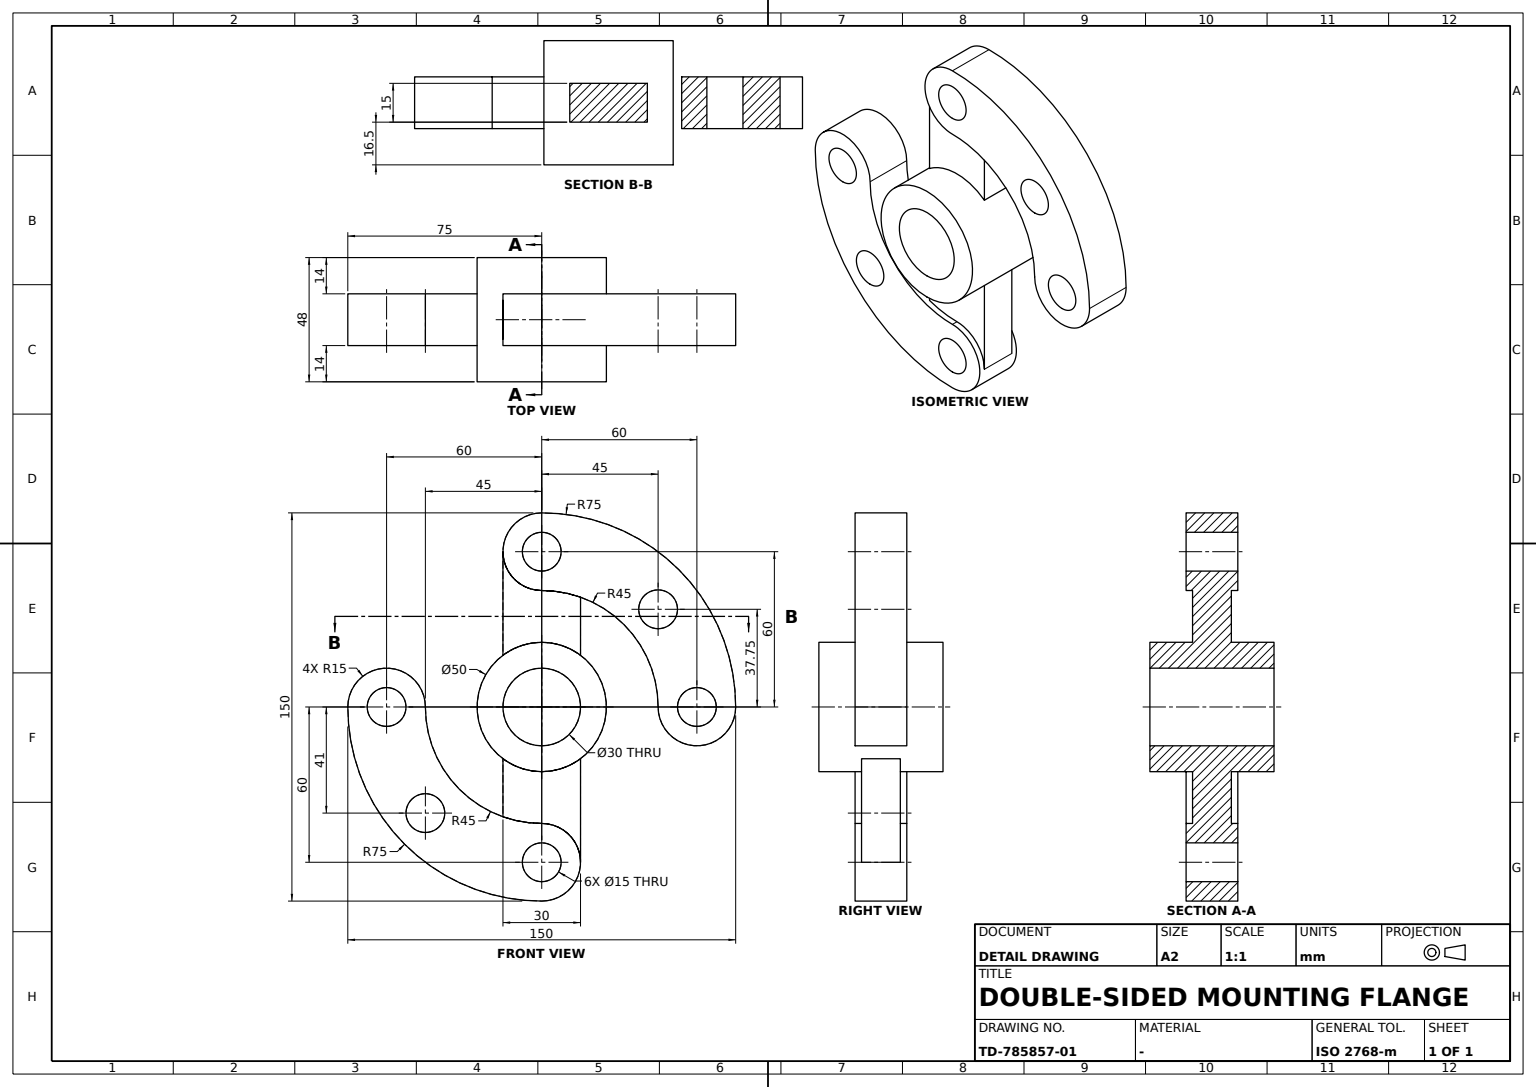
ISO-10303-21;
HEADER;
FILE_DESCRIPTION((''),'2;1');
FILE_NAME('','',(''),(''),'','','');
FILE_SCHEMA(('AUTOMOTIVE_DESIGN'));
ENDSEC;
DATA;
#1=APPLICATION_CONTEXT('');
#2=PRODUCT_CONTEXT('',#1,'mechanical');
#3=PRODUCT('','','',(#2));
#4=PRODUCT_DEFINITION_FORMATION('','',#3);
#5=PRODUCT_DEFINITION_CONTEXT('',#1,'design');
#6=PRODUCT_DEFINITION('','',#4,#5);
#7=PRODUCT_DEFINITION_SHAPE('','',#6);
#8=(LENGTH_UNIT()NAMED_UNIT(*)SI_UNIT(.MILLI.,.METRE.));
#9=(NAMED_UNIT(*)PLANE_ANGLE_UNIT()SI_UNIT($,.RADIAN.));
#10=(NAMED_UNIT(*)SI_UNIT($,.STERADIAN.)SOLID_ANGLE_UNIT());
#11=UNCERTAINTY_MEASURE_WITH_UNIT(LENGTH_MEASURE(0.005),#8,'distance_accuracy_value','');
#12=(GEOMETRIC_REPRESENTATION_CONTEXT(3)GLOBAL_UNCERTAINTY_ASSIGNED_CONTEXT((#11))GLOBAL_UNIT_ASSIGNED_CONTEXT((#8,#9,#10))REPRESENTATION_CONTEXT('',''));
#13=CARTESIAN_POINT('',(-10.,-60.,-7.5));
#14=VERTEX_POINT('',#13);
#15=CARTESIAN_POINT('',(-10.,-60.,0.));
#16=DIRECTION('',(1.,0.,0.));
#17=DIRECTION('',(0.,0.,-1.));
#18=AXIS2_PLACEMENT_3D('',#15,#16,#17);
#19=CIRCLE('',#18,7.5);
#20=EDGE_CURVE('',#14,#14,#19,.T.);
#21=ORIENTED_EDGE('',*,*,#20,.F.);
#22=EDGE_LOOP('',(#21));
#23=FACE_BOUND('',#22,.T.);
#24=CARTESIAN_POINT('',(10.,-60.,-7.5));
#25=VERTEX_POINT('',#24);
#26=CARTESIAN_POINT('',(10.,-60.,0.));
#27=AXIS2_PLACEMENT_3D('',#26,#16,#17);
#28=CIRCLE('',#27,7.5);
#29=EDGE_CURVE('',#25,#25,#28,.T.);
#30=ORIENTED_EDGE('',*,*,#29,.T.);
#31=EDGE_LOOP('',(#30));
#32=FACE_BOUND('',#31,.T.);
#33=CARTESIAN_POINT('',(0.,-60.,0.));
#34=DIRECTION('',(0.,1.,0.));
#35=AXIS2_PLACEMENT_3D('',#33,#16,#34);
#36=CYLINDRICAL_SURFACE('',#35,7.5);
#37=ADVANCED_FACE('',(#23,#32),#36,.F.);
#38=CARTESIAN_POINT('',(-10.,-45.,-48.498329));
#39=VERTEX_POINT('',#38);
#40=CARTESIAN_POINT('',(-10.,-45.,-40.998329));
#41=AXIS2_PLACEMENT_3D('',#40,#16,#17);
#42=CIRCLE('',#41,7.5);
#43=EDGE_CURVE('',#39,#39,#42,.T.);
#44=ORIENTED_EDGE('',*,*,#43,.T.);
#45=EDGE_LOOP('',(#44));
#46=FACE_BOUND('',#45,.T.);
#47=CARTESIAN_POINT('',(-10.,0.,-67.5));
#48=VERTEX_POINT('',#47);
#49=CARTESIAN_POINT('',(-10.,0.,-60.));
#50=AXIS2_PLACEMENT_3D('',#49,#16,#17);
#51=CIRCLE('',#50,7.5);
#52=EDGE_CURVE('',#48,#48,#51,.T.);
#53=ORIENTED_EDGE('',*,*,#52,.T.);
#54=EDGE_LOOP('',(#53));
#55=FACE_BOUND('',#54,.T.);
#56=CARTESIAN_POINT('',(-10.,-45.,0.));
#57=VERTEX_POINT('',#56);
#58=CARTESIAN_POINT('',(-10.,0.,-45.));
#59=VERTEX_POINT('',#58);
#60=CARTESIAN_POINT('',(-10.,0.,0.));
#61=AXIS2_PLACEMENT_3D('',#60,#16,#17);
#62=CIRCLE('',#61,45.);
#63=EDGE_CURVE('',#57,#59,#62,.T.);
#64=ORIENTED_EDGE('',*,*,#63,.T.);
#65=CARTESIAN_POINT('',(-10.,0.,-75.));
#66=VERTEX_POINT('',#65);
#67=CIRCLE('',#50,15.);
#68=EDGE_CURVE('',#66,#59,#67,.T.);
#69=ORIENTED_EDGE('',*,*,#68,.F.);
#70=CARTESIAN_POINT('',(-10.,-75.,0.));
#71=VERTEX_POINT('',#70);
#72=CIRCLE('',#61,75.);
#73=EDGE_CURVE('',#71,#66,#72,.T.);
#74=ORIENTED_EDGE('',*,*,#73,.F.);
#75=CIRCLE('',#18,15.);
#76=EDGE_CURVE('',#57,#71,#75,.T.);
#77=ORIENTED_EDGE('',*,*,#76,.F.);
#78=EDGE_LOOP('',(#64,#69,#74,#77));
#79=FACE_BOUND('',#78,.T.);
#80=ORIENTED_EDGE('',*,*,#20,.T.);
#81=EDGE_LOOP('',(#80));
#82=FACE_BOUND('',#81,.T.);
#83=AXIS2_PLACEMENT_3D('',#60,#16,#34);
#84=PLANE('',#83);
#85=ADVANCED_FACE('',(#46,#55,#79,#82),#84,.F.);
#86=CARTESIAN_POINT('',(-10.,60.,-7.5));
#87=VERTEX_POINT('',#86);
#88=CARTESIAN_POINT('',(-10.,60.,0.));
#89=AXIS2_PLACEMENT_3D('',#88,#16,#17);
#90=CIRCLE('',#89,7.5);
#91=EDGE_CURVE('',#87,#87,#90,.T.);
#92=ORIENTED_EDGE('',*,*,#91,.F.);
#93=EDGE_LOOP('',(#92));
#94=FACE_BOUND('',#93,.T.);
#95=CARTESIAN_POINT('',(10.,60.,-7.5));
#96=VERTEX_POINT('',#95);
#97=CARTESIAN_POINT('',(10.,60.,0.));
#98=AXIS2_PLACEMENT_3D('',#97,#16,#17);
#99=CIRCLE('',#98,7.5);
#100=EDGE_CURVE('',#96,#96,#99,.T.);
#101=ORIENTED_EDGE('',*,*,#100,.T.);
#102=EDGE_LOOP('',(#101));
#103=FACE_BOUND('',#102,.T.);
#104=CARTESIAN_POINT('',(0.,60.,0.));
#105=AXIS2_PLACEMENT_3D('',#104,#16,#34);
#106=CYLINDRICAL_SURFACE('',#105,7.5);
#107=ADVANCED_FACE('',(#94,#103),#106,.F.);
#108=CARTESIAN_POINT('',(24.,0.,-25.));
#109=VERTEX_POINT('',#108);
#110=CARTESIAN_POINT('',(24.,0.,0.));
#111=AXIS2_PLACEMENT_3D('',#110,#16,#17);
#112=CIRCLE('',#111,25.);
#113=EDGE_CURVE('',#109,#109,#112,.T.);
#114=ORIENTED_EDGE('',*,*,#113,.F.);
#115=EDGE_LOOP('',(#114));
#116=FACE_BOUND('',#115,.T.);
#117=CARTESIAN_POINT('',(-7.5,15.,20.));
#118=VERTEX_POINT('',#117);
#119=CARTESIAN_POINT('',(-7.5,-15.,20.));
#120=VERTEX_POINT('',#119);
#121=CARTESIAN_POINT('',(-7.5,0.,0.));
#122=AXIS2_PLACEMENT_3D('',#121,#16,#17);
#123=CIRCLE('',#122,25.);
#124=EDGE_CURVE('',#118,#120,#123,.T.);
#125=ORIENTED_EDGE('',*,*,#124,.F.);
#126=CARTESIAN_POINT('',(7.5,15.,20.));
#127=VERTEX_POINT('',#126);
#128=VECTOR('',#16,1000.);
#129=LINE('',#117,#128);
#130=EDGE_CURVE('',#118,#127,#129,.T.);
#131=ORIENTED_EDGE('',*,*,#130,.T.);
#132=CARTESIAN_POINT('',(7.5,-15.,20.));
#133=VERTEX_POINT('',#132);
#134=CARTESIAN_POINT('',(7.5,0.,0.));
#135=AXIS2_PLACEMENT_3D('',#134,#16,#17);
#136=CIRCLE('',#135,25.);
#137=EDGE_CURVE('',#127,#133,#136,.T.);
#138=ORIENTED_EDGE('',*,*,#137,.T.);
#139=LINE('',#119,#128);
#140=EDGE_CURVE('',#120,#133,#139,.T.);
#141=ORIENTED_EDGE('',*,*,#140,.F.);
#142=EDGE_LOOP('',(#125,#131,#138,#141));
#143=FACE_BOUND('',#142,.T.);
#144=CARTESIAN_POINT('',(-7.5,-15.,-20.));
#145=VERTEX_POINT('',#144);
#146=CARTESIAN_POINT('',(7.5,-15.,-20.));
#147=VERTEX_POINT('',#146);
#148=LINE('',#144,#128);
#149=EDGE_CURVE('',#145,#147,#148,.T.);
#150=ORIENTED_EDGE('',*,*,#149,.T.);
#151=CARTESIAN_POINT('',(7.5,15.,-20.));
#152=VERTEX_POINT('',#151);
#153=EDGE_CURVE('',#147,#152,#136,.T.);
#154=ORIENTED_EDGE('',*,*,#153,.T.);
#155=CARTESIAN_POINT('',(-7.5,15.,-20.));
#156=VERTEX_POINT('',#155);
#157=LINE('',#155,#128);
#158=EDGE_CURVE('',#156,#152,#157,.T.);
#159=ORIENTED_EDGE('',*,*,#158,.F.);
#160=EDGE_CURVE('',#145,#156,#123,.T.);
#161=ORIENTED_EDGE('',*,*,#160,.F.);
#162=EDGE_LOOP('',(#150,#154,#159,#161));
#163=FACE_BOUND('',#162,.T.);
#164=CARTESIAN_POINT('',(-24.,0.,-25.));
#165=VERTEX_POINT('',#164);
#166=CARTESIAN_POINT('',(-24.,0.,0.));
#167=AXIS2_PLACEMENT_3D('',#166,#16,#17);
#168=CIRCLE('',#167,25.);
#169=EDGE_CURVE('',#165,#165,#168,.T.);
#170=ORIENTED_EDGE('',*,*,#169,.T.);
#171=EDGE_LOOP('',(#170));
#172=FACE_BOUND('',#171,.T.);
#173=CARTESIAN_POINT('',(0.,0.,0.));
#174=AXIS2_PLACEMENT_3D('',#173,#16,#34);
#175=CYLINDRICAL_SURFACE('',#174,25.);
#176=ADVANCED_FACE('',(#116,#143,#163,#172),#175,.T.);
#177=CARTESIAN_POINT('',(7.5,15.,42.426407));
#178=VERTEX_POINT('',#177);
#179=CARTESIAN_POINT('',(7.5,0.,45.));
#180=VERTEX_POINT('',#179);
#181=CIRCLE('',#135,45.);
#182=EDGE_CURVE('',#178,#180,#181,.T.);
#183=ORIENTED_EDGE('',*,*,#182,.T.);
#184=CARTESIAN_POINT('',(7.5,-15.,60.));
#185=VERTEX_POINT('',#184);
#186=CARTESIAN_POINT('',(7.5,0.,60.));
#187=AXIS2_PLACEMENT_3D('',#186,#16,#17);
#188=CIRCLE('',#187,15.);
#189=EDGE_CURVE('',#185,#180,#188,.T.);
#190=ORIENTED_EDGE('',*,*,#189,.F.);
#191=CARTESIAN_POINT('',(7.5,-15.,0.));
#192=DIRECTION('',(0.,0.,1.));
#193=VECTOR('',#192,1000.);
#194=LINE('',#191,#193);
#195=EDGE_CURVE('',#133,#185,#194,.T.);
#196=ORIENTED_EDGE('',*,*,#195,.F.);
#197=ORIENTED_EDGE('',*,*,#137,.F.);
#198=CARTESIAN_POINT('',(7.5,15.,0.));
#199=VECTOR('',#17,1000.);
#200=LINE('',#198,#199);
#201=EDGE_CURVE('',#178,#127,#200,.T.);
#202=ORIENTED_EDGE('',*,*,#201,.F.);
#203=EDGE_LOOP('',(#183,#190,#196,#197,#202));
#204=FACE_BOUND('',#203,.T.);
#205=AXIS2_PLACEMENT_3D('',#134,#16,#34);
#206=PLANE('',#205);
#207=ADVANCED_FACE('',(#204),#206,.T.);
#208=CARTESIAN_POINT('',(7.5,15.,-60.));
#209=VERTEX_POINT('',#208);
#210=CARTESIAN_POINT('',(7.5,0.,-45.));
#211=VERTEX_POINT('',#210);
#212=CARTESIAN_POINT('',(7.5,0.,-60.));
#213=AXIS2_PLACEMENT_3D('',#212,#16,#17);
#214=CIRCLE('',#213,15.);
#215=EDGE_CURVE('',#209,#211,#214,.T.);
#216=ORIENTED_EDGE('',*,*,#215,.F.);
#217=CARTESIAN_POINT('',(7.5,15.,75.));
#218=LINE('',#217,#193);
#219=EDGE_CURVE('',#209,#152,#218,.T.);
#220=ORIENTED_EDGE('',*,*,#219,.T.);
#221=ORIENTED_EDGE('',*,*,#153,.F.);
#222=CARTESIAN_POINT('',(7.5,-15.,-42.426407));
#223=VERTEX_POINT('',#222);
#224=LINE('',#132,#199);
#225=EDGE_CURVE('',#147,#223,#224,.T.);
#226=ORIENTED_EDGE('',*,*,#225,.T.);
#227=EDGE_CURVE('',#223,#211,#181,.T.);
#228=ORIENTED_EDGE('',*,*,#227,.T.);
#229=EDGE_LOOP('',(#216,#220,#221,#226,#228));
#230=FACE_BOUND('',#229,.T.);
#231=ADVANCED_FACE('',(#230),#206,.T.);
#232=CARTESIAN_POINT('',(10.,45.,0.));
#233=VERTEX_POINT('',#232);
#234=CARTESIAN_POINT('',(10.,75.,0.));
#235=VERTEX_POINT('',#234);
#236=CIRCLE('',#98,15.);
#237=EDGE_CURVE('',#233,#235,#236,.T.);
#238=ORIENTED_EDGE('',*,*,#237,.F.);
#239=CARTESIAN_POINT('',(-10.,45.,0.));
#240=VERTEX_POINT('',#239);
#241=CARTESIAN_POINT('',(0.,45.,0.));
#242=LINE('',#241,#128);
#243=EDGE_CURVE('',#240,#233,#242,.T.);
#244=ORIENTED_EDGE('',*,*,#243,.F.);
#245=CARTESIAN_POINT('',(-10.,75.,0.));
#246=VERTEX_POINT('',#245);
#247=CIRCLE('',#89,15.);
#248=EDGE_CURVE('',#240,#246,#247,.T.);
#249=ORIENTED_EDGE('',*,*,#248,.T.);
#250=CARTESIAN_POINT('',(0.,75.,0.));
#251=LINE('',#250,#128);
#252=EDGE_CURVE('',#246,#235,#251,.T.);
#253=ORIENTED_EDGE('',*,*,#252,.T.);
#254=EDGE_LOOP('',(#238,#244,#249,#253));
#255=FACE_BOUND('',#254,.T.);
#256=CYLINDRICAL_SURFACE('',#105,15.);
#257=ADVANCED_FACE('',(#255),#256,.T.);
#258=CARTESIAN_POINT('',(-7.5,-15.,60.));
#259=VERTEX_POINT('',#258);
#260=CARTESIAN_POINT('',(0.,-15.,60.));
#261=LINE('',#260,#128);
#262=EDGE_CURVE('',#259,#185,#261,.T.);
#263=ORIENTED_EDGE('',*,*,#262,.F.);
#264=CARTESIAN_POINT('',(-7.5,-15.,0.));
#265=LINE('',#264,#193);
#266=EDGE_CURVE('',#120,#259,#265,.T.);
#267=ORIENTED_EDGE('',*,*,#266,.F.);
#268=ORIENTED_EDGE('',*,*,#140,.T.);
#269=ORIENTED_EDGE('',*,*,#195,.T.);
#270=EDGE_LOOP('',(#263,#267,#268,#269));
#271=FACE_BOUND('',#270,.T.);
#272=CARTESIAN_POINT('',(0.,-15.,20.));
#273=AXIS2_PLACEMENT_3D('',#272,#34,#192);
#274=PLANE('',#273);
#275=ADVANCED_FACE('',(#271),#274,.F.);
#276=CARTESIAN_POINT('',(10.,0.,-75.));
#277=VERTEX_POINT('',#276);
#278=CARTESIAN_POINT('',(10.,0.,-45.));
#279=VERTEX_POINT('',#278);
#280=CARTESIAN_POINT('',(10.,0.,-60.));
#281=AXIS2_PLACEMENT_3D('',#280,#16,#17);
#282=CIRCLE('',#281,15.);
#283=EDGE_CURVE('',#277,#279,#282,.T.);
#284=ORIENTED_EDGE('',*,*,#283,.T.);
#285=CARTESIAN_POINT('',(10.,-45.,0.));
#286=VERTEX_POINT('',#285);
#287=CARTESIAN_POINT('',(10.,0.,0.));
#288=AXIS2_PLACEMENT_3D('',#287,#16,#17);
#289=CIRCLE('',#288,45.);
#290=EDGE_CURVE('',#286,#279,#289,.T.);
#291=ORIENTED_EDGE('',*,*,#290,.F.);
#292=CARTESIAN_POINT('',(10.,-75.,0.));
#293=VERTEX_POINT('',#292);
#294=CIRCLE('',#27,15.);
#295=EDGE_CURVE('',#286,#293,#294,.T.);
#296=ORIENTED_EDGE('',*,*,#295,.T.);
#297=CIRCLE('',#288,75.);
#298=EDGE_CURVE('',#293,#277,#297,.T.);
#299=ORIENTED_EDGE('',*,*,#298,.T.);
#300=EDGE_LOOP('',(#284,#291,#296,#299));
#301=FACE_BOUND('',#300,.T.);
#302=ORIENTED_EDGE('',*,*,#29,.F.);
#303=EDGE_LOOP('',(#302));
#304=FACE_BOUND('',#303,.T.);
#305=CARTESIAN_POINT('',(10.,0.,-67.5));
#306=VERTEX_POINT('',#305);
#307=CIRCLE('',#281,7.5);
#308=EDGE_CURVE('',#306,#306,#307,.T.);
#309=ORIENTED_EDGE('',*,*,#308,.F.);
#310=EDGE_LOOP('',(#309));
#311=FACE_BOUND('',#310,.T.);
#312=CARTESIAN_POINT('',(10.,-45.,-48.498329));
#313=VERTEX_POINT('',#312);
#314=CARTESIAN_POINT('',(10.,-45.,-40.998329));
#315=AXIS2_PLACEMENT_3D('',#314,#16,#17);
#316=CIRCLE('',#315,7.5);
#317=EDGE_CURVE('',#313,#313,#316,.T.);
#318=ORIENTED_EDGE('',*,*,#317,.F.);
#319=EDGE_LOOP('',(#318));
#320=FACE_BOUND('',#319,.T.);
#321=AXIS2_PLACEMENT_3D('',#287,#16,#34);
#322=PLANE('',#321);
#323=ADVANCED_FACE('',(#301,#304,#311,#320),#322,.T.);
#324=ORIENTED_EDGE('',*,*,#52,.F.);
#325=EDGE_LOOP('',(#324));
#326=FACE_BOUND('',#325,.T.);
#327=ORIENTED_EDGE('',*,*,#308,.T.);
#328=EDGE_LOOP('',(#327));
#329=FACE_BOUND('',#328,.T.);
#330=CARTESIAN_POINT('',(0.,0.,-60.));
#331=AXIS2_PLACEMENT_3D('',#330,#16,#34);
#332=CYLINDRICAL_SURFACE('',#331,7.5);
#333=ADVANCED_FACE('',(#326,#329),#332,.F.);
#334=ORIENTED_EDGE('',*,*,#215,.T.);
#335=CARTESIAN_POINT('',(8.75,0.,-45.));
#336=LINE('',#335,#128);
#337=EDGE_CURVE('',#211,#279,#336,.T.);
#338=ORIENTED_EDGE('',*,*,#337,.T.);
#339=ORIENTED_EDGE('',*,*,#283,.F.);
#340=CARTESIAN_POINT('',(0.,0.,-75.));
#341=LINE('',#340,#128);
#342=EDGE_CURVE('',#66,#277,#341,.T.);
#343=ORIENTED_EDGE('',*,*,#342,.F.);
#344=ORIENTED_EDGE('',*,*,#68,.T.);
#345=CARTESIAN_POINT('',(-7.5,0.,-45.));
#346=VERTEX_POINT('',#345);
#347=CARTESIAN_POINT('',(-8.75,0.,-45.));
#348=LINE('',#347,#128);
#349=EDGE_CURVE('',#59,#346,#348,.T.);
#350=ORIENTED_EDGE('',*,*,#349,.T.);
#351=CARTESIAN_POINT('',(-7.5,15.,-60.));
#352=VERTEX_POINT('',#351);
#353=CARTESIAN_POINT('',(-7.5,0.,-60.));
#354=AXIS2_PLACEMENT_3D('',#353,#16,#17);
#355=CIRCLE('',#354,15.);
#356=EDGE_CURVE('',#352,#346,#355,.T.);
#357=ORIENTED_EDGE('',*,*,#356,.F.);
#358=CARTESIAN_POINT('',(0.,15.,-60.));
#359=LINE('',#358,#128);
#360=EDGE_CURVE('',#352,#209,#359,.T.);
#361=ORIENTED_EDGE('',*,*,#360,.T.);
#362=EDGE_LOOP('',(#334,#338,#339,#343,#344,#350,#357,#361));
#363=FACE_BOUND('',#362,.T.);
#364=CYLINDRICAL_SURFACE('',#331,15.);
#365=ADVANCED_FACE('',(#363),#364,.T.);
#366=ORIENTED_EDGE('',*,*,#290,.T.);
#367=ORIENTED_EDGE('',*,*,#337,.F.);
#368=ORIENTED_EDGE('',*,*,#227,.F.);
#369=CARTESIAN_POINT('',(-7.5,-15.,-42.426407));
#370=VERTEX_POINT('',#369);
#371=LINE('',#369,#128);
#372=EDGE_CURVE('',#370,#223,#371,.T.);
#373=ORIENTED_EDGE('',*,*,#372,.F.);
#374=CIRCLE('',#122,45.);
#375=EDGE_CURVE('',#370,#346,#374,.T.);
#376=ORIENTED_EDGE('',*,*,#375,.T.);
#377=ORIENTED_EDGE('',*,*,#349,.F.);
#378=ORIENTED_EDGE('',*,*,#63,.F.);
#379=CARTESIAN_POINT('',(0.,-45.,0.));
#380=LINE('',#379,#128);
#381=EDGE_CURVE('',#57,#286,#380,.T.);
#382=ORIENTED_EDGE('',*,*,#381,.T.);
#383=EDGE_LOOP('',(#366,#367,#368,#373,#376,#377,#378,#382));
#384=FACE_BOUND('',#383,.T.);
#385=CYLINDRICAL_SURFACE('',#174,45.);
#386=ADVANCED_FACE('',(#384),#385,.F.);
#387=ORIENTED_EDGE('',*,*,#130,.F.);
#388=CARTESIAN_POINT('',(-7.5,15.,42.426407));
#389=VERTEX_POINT('',#388);
#390=CARTESIAN_POINT('',(-7.5,15.,0.));
#391=LINE('',#390,#199);
#392=EDGE_CURVE('',#389,#118,#391,.T.);
#393=ORIENTED_EDGE('',*,*,#392,.F.);
#394=LINE('',#388,#128);
#395=EDGE_CURVE('',#389,#178,#394,.T.);
#396=ORIENTED_EDGE('',*,*,#395,.T.);
#397=ORIENTED_EDGE('',*,*,#201,.T.);
#398=EDGE_LOOP('',(#387,#393,#396,#397));
#399=FACE_BOUND('',#398,.T.);
#400=CARTESIAN_POINT('',(0.,15.,75.));
#401=DIRECTION('',(0.,-1.,0.));
#402=AXIS2_PLACEMENT_3D('',#400,#401,#17);
#403=PLANE('',#402);
#404=ADVANCED_FACE('',(#399),#403,.F.);
#405=CARTESIAN_POINT('',(-10.,0.,52.5));
#406=VERTEX_POINT('',#405);
#407=CARTESIAN_POINT('',(-10.,0.,60.));
#408=AXIS2_PLACEMENT_3D('',#407,#16,#17);
#409=CIRCLE('',#408,7.5);
#410=EDGE_CURVE('',#406,#406,#409,.T.);
#411=ORIENTED_EDGE('',*,*,#410,.F.);
#412=EDGE_LOOP('',(#411));
#413=FACE_BOUND('',#412,.T.);
#414=CARTESIAN_POINT('',(10.,0.,52.5));
#415=VERTEX_POINT('',#414);
#416=CARTESIAN_POINT('',(10.,0.,60.));
#417=AXIS2_PLACEMENT_3D('',#416,#16,#17);
#418=CIRCLE('',#417,7.5);
#419=EDGE_CURVE('',#415,#415,#418,.T.);
#420=ORIENTED_EDGE('',*,*,#419,.T.);
#421=EDGE_LOOP('',(#420));
#422=FACE_BOUND('',#421,.T.);
#423=CARTESIAN_POINT('',(0.,0.,60.));
#424=AXIS2_PLACEMENT_3D('',#423,#16,#34);
#425=CYLINDRICAL_SURFACE('',#424,7.5);
#426=ADVANCED_FACE('',(#413,#422),#425,.F.);
#427=CARTESIAN_POINT('',(10.,45.,30.24617));
#428=VERTEX_POINT('',#427);
#429=CARTESIAN_POINT('',(10.,45.,37.74617));
#430=AXIS2_PLACEMENT_3D('',#429,#16,#17);
#431=CIRCLE('',#430,7.5);
#432=EDGE_CURVE('',#428,#428,#431,.T.);
#433=ORIENTED_EDGE('',*,*,#432,.T.);
#434=EDGE_LOOP('',(#433));
#435=FACE_BOUND('',#434,.T.);
#436=CARTESIAN_POINT('',(-10.,45.,30.24617));
#437=VERTEX_POINT('',#436);
#438=CARTESIAN_POINT('',(-10.,45.,37.74617));
#439=AXIS2_PLACEMENT_3D('',#438,#16,#17);
#440=CIRCLE('',#439,7.5);
#441=EDGE_CURVE('',#437,#437,#440,.T.);
#442=ORIENTED_EDGE('',*,*,#441,.F.);
#443=EDGE_LOOP('',(#442));
#444=FACE_BOUND('',#443,.T.);
#445=CARTESIAN_POINT('',(0.,45.,37.74617));
#446=AXIS2_PLACEMENT_3D('',#445,#16,#34);
#447=CYLINDRICAL_SURFACE('',#446,7.5);
#448=ADVANCED_FACE('',(#435,#444),#447,.F.);
#449=CARTESIAN_POINT('',(24.,0.,-15.));
#450=VERTEX_POINT('',#449);
#451=CIRCLE('',#111,15.);
#452=EDGE_CURVE('',#450,#450,#451,.T.);
#453=ORIENTED_EDGE('',*,*,#452,.T.);
#454=EDGE_LOOP('',(#453));
#455=FACE_BOUND('',#454,.T.);
#456=CARTESIAN_POINT('',(-24.,0.,-15.));
#457=VERTEX_POINT('',#456);
#458=CIRCLE('',#167,15.);
#459=EDGE_CURVE('',#457,#457,#458,.T.);
#460=ORIENTED_EDGE('',*,*,#459,.F.);
#461=EDGE_LOOP('',(#460));
#462=FACE_BOUND('',#461,.T.);
#463=CYLINDRICAL_SURFACE('',#174,15.);
#464=ADVANCED_FACE('',(#455,#462),#463,.F.);
#465=ORIENTED_EDGE('',*,*,#317,.T.);
#466=EDGE_LOOP('',(#465));
#467=FACE_BOUND('',#466,.T.);
#468=ORIENTED_EDGE('',*,*,#43,.F.);
#469=EDGE_LOOP('',(#468));
#470=FACE_BOUND('',#469,.T.);
#471=CARTESIAN_POINT('',(0.,-45.,-40.998329));
#472=AXIS2_PLACEMENT_3D('',#471,#16,#34);
#473=CYLINDRICAL_SURFACE('',#472,7.5);
#474=ADVANCED_FACE('',(#467,#470),#473,.F.);
#475=CARTESIAN_POINT('',(-7.5,0.,45.));
#476=VERTEX_POINT('',#475);
#477=EDGE_CURVE('',#389,#476,#374,.T.);
#478=ORIENTED_EDGE('',*,*,#477,.F.);
#479=ORIENTED_EDGE('',*,*,#392,.T.);
#480=ORIENTED_EDGE('',*,*,#124,.T.);
#481=ORIENTED_EDGE('',*,*,#266,.T.);
#482=CARTESIAN_POINT('',(-7.5,0.,60.));
#483=AXIS2_PLACEMENT_3D('',#482,#16,#17);
#484=CIRCLE('',#483,15.);
#485=EDGE_CURVE('',#259,#476,#484,.T.);
#486=ORIENTED_EDGE('',*,*,#485,.T.);
#487=EDGE_LOOP('',(#478,#479,#480,#481,#486));
#488=FACE_BOUND('',#487,.T.);
#489=AXIS2_PLACEMENT_3D('',#121,#16,#34);
#490=PLANE('',#489);
#491=ADVANCED_FACE('',(#488),#490,.F.);
#492=ORIENTED_EDGE('',*,*,#160,.T.);
#493=CARTESIAN_POINT('',(-7.5,15.,75.));
#494=LINE('',#493,#193);
#495=EDGE_CURVE('',#352,#156,#494,.T.);
#496=ORIENTED_EDGE('',*,*,#495,.F.);
#497=ORIENTED_EDGE('',*,*,#356,.T.);
#498=ORIENTED_EDGE('',*,*,#375,.F.);
#499=LINE('',#119,#199);
#500=EDGE_CURVE('',#145,#370,#499,.T.);
#501=ORIENTED_EDGE('',*,*,#500,.F.);
#502=EDGE_LOOP('',(#492,#496,#497,#498,#501));
#503=FACE_BOUND('',#502,.T.);
#504=ADVANCED_FACE('',(#503),#490,.F.);
#505=CARTESIAN_POINT('',(0.,-75.,0.));
#506=LINE('',#505,#128);
#507=EDGE_CURVE('',#71,#293,#506,.T.);
#508=ORIENTED_EDGE('',*,*,#507,.F.);
#509=ORIENTED_EDGE('',*,*,#73,.T.);
#510=ORIENTED_EDGE('',*,*,#342,.T.);
#511=ORIENTED_EDGE('',*,*,#298,.F.);
#512=EDGE_LOOP('',(#508,#509,#510,#511));
#513=FACE_BOUND('',#512,.T.);
#514=CYLINDRICAL_SURFACE('',#174,75.);
#515=ADVANCED_FACE('',(#513),#514,.T.);
#516=CARTESIAN_POINT('',(10.,0.,75.));
#517=VERTEX_POINT('',#516);
#518=EDGE_CURVE('',#235,#517,#297,.T.);
#519=ORIENTED_EDGE('',*,*,#518,.F.);
#520=ORIENTED_EDGE('',*,*,#252,.F.);
#521=CARTESIAN_POINT('',(-10.,0.,75.));
#522=VERTEX_POINT('',#521);
#523=EDGE_CURVE('',#246,#522,#72,.T.);
#524=ORIENTED_EDGE('',*,*,#523,.T.);
#525=CARTESIAN_POINT('',(0.,0.,75.));
#526=LINE('',#525,#128);
#527=EDGE_CURVE('',#522,#517,#526,.T.);
#528=ORIENTED_EDGE('',*,*,#527,.T.);
#529=EDGE_LOOP('',(#519,#520,#524,#528));
#530=FACE_BOUND('',#529,.T.);
#531=ADVANCED_FACE('',(#530),#514,.T.);
#532=ORIENTED_EDGE('',*,*,#225,.F.);
#533=ORIENTED_EDGE('',*,*,#149,.F.);
#534=ORIENTED_EDGE('',*,*,#500,.T.);
#535=ORIENTED_EDGE('',*,*,#372,.T.);
#536=EDGE_LOOP('',(#532,#533,#534,#535));
#537=FACE_BOUND('',#536,.T.);
#538=ADVANCED_FACE('',(#537),#274,.F.);
#539=ORIENTED_EDGE('',*,*,#113,.T.);
#540=EDGE_LOOP('',(#539));
#541=FACE_BOUND('',#540,.T.);
#542=ORIENTED_EDGE('',*,*,#452,.F.);
#543=EDGE_LOOP('',(#542));
#544=FACE_BOUND('',#543,.T.);
#545=AXIS2_PLACEMENT_3D('',#110,#16,#34);
#546=PLANE('',#545);
#547=ADVANCED_FACE('',(#541,#544),#546,.T.);
#548=ORIENTED_EDGE('',*,*,#169,.F.);
#549=EDGE_LOOP('',(#548));
#550=FACE_BOUND('',#549,.T.);
#551=ORIENTED_EDGE('',*,*,#459,.T.);
#552=EDGE_LOOP('',(#551));
#553=FACE_BOUND('',#552,.T.);
#554=AXIS2_PLACEMENT_3D('',#166,#16,#34);
#555=PLANE('',#554);
#556=ADVANCED_FACE('',(#550,#553),#555,.F.);
#557=ORIENTED_EDGE('',*,*,#518,.T.);
#558=CARTESIAN_POINT('',(10.,0.,45.));
#559=VERTEX_POINT('',#558);
#560=CIRCLE('',#417,15.);
#561=EDGE_CURVE('',#517,#559,#560,.T.);
#562=ORIENTED_EDGE('',*,*,#561,.T.);
#563=EDGE_CURVE('',#233,#559,#289,.T.);
#564=ORIENTED_EDGE('',*,*,#563,.F.);
#565=ORIENTED_EDGE('',*,*,#237,.T.);
#566=EDGE_LOOP('',(#557,#562,#564,#565));
#567=FACE_BOUND('',#566,.T.);
#568=ORIENTED_EDGE('',*,*,#100,.F.);
#569=EDGE_LOOP('',(#568));
#570=FACE_BOUND('',#569,.T.);
#571=ORIENTED_EDGE('',*,*,#419,.F.);
#572=EDGE_LOOP('',(#571));
#573=FACE_BOUND('',#572,.T.);
#574=ORIENTED_EDGE('',*,*,#432,.F.);
#575=EDGE_LOOP('',(#574));
#576=FACE_BOUND('',#575,.T.);
#577=ADVANCED_FACE('',(#567,#570,#573,#576),#322,.T.);
#578=ORIENTED_EDGE('',*,*,#507,.T.);
#579=ORIENTED_EDGE('',*,*,#295,.F.);
#580=ORIENTED_EDGE('',*,*,#381,.F.);
#581=ORIENTED_EDGE('',*,*,#76,.T.);
#582=EDGE_LOOP('',(#578,#579,#580,#581));
#583=FACE_BOUND('',#582,.T.);
#584=CYLINDRICAL_SURFACE('',#35,15.);
#585=ADVANCED_FACE('',(#583),#584,.T.);
#586=ORIENTED_EDGE('',*,*,#495,.T.);
#587=ORIENTED_EDGE('',*,*,#158,.T.);
#588=ORIENTED_EDGE('',*,*,#219,.F.);
#589=ORIENTED_EDGE('',*,*,#360,.F.);
#590=EDGE_LOOP('',(#586,#587,#588,#589));
#591=FACE_BOUND('',#590,.T.);
#592=ADVANCED_FACE('',(#591),#403,.F.);
#593=ORIENTED_EDGE('',*,*,#91,.T.);
#594=EDGE_LOOP('',(#593));
#595=FACE_BOUND('',#594,.T.);
#596=ORIENTED_EDGE('',*,*,#441,.T.);
#597=EDGE_LOOP('',(#596));
#598=FACE_BOUND('',#597,.T.);
#599=ORIENTED_EDGE('',*,*,#248,.F.);
#600=CARTESIAN_POINT('',(-10.,0.,45.));
#601=VERTEX_POINT('',#600);
#602=EDGE_CURVE('',#240,#601,#62,.T.);
#603=ORIENTED_EDGE('',*,*,#602,.T.);
#604=CIRCLE('',#408,15.);
#605=EDGE_CURVE('',#522,#601,#604,.T.);
#606=ORIENTED_EDGE('',*,*,#605,.F.);
#607=ORIENTED_EDGE('',*,*,#523,.F.);
#608=EDGE_LOOP('',(#599,#603,#606,#607));
#609=FACE_BOUND('',#608,.T.);
#610=ORIENTED_EDGE('',*,*,#410,.T.);
#611=EDGE_LOOP('',(#610));
#612=FACE_BOUND('',#611,.T.);
#613=ADVANCED_FACE('',(#595,#598,#609,#612),#84,.F.);
#614=ORIENTED_EDGE('',*,*,#485,.F.);
#615=ORIENTED_EDGE('',*,*,#262,.T.);
#616=ORIENTED_EDGE('',*,*,#189,.T.);
#617=CARTESIAN_POINT('',(8.75,0.,45.));
#618=LINE('',#617,#128);
#619=EDGE_CURVE('',#180,#559,#618,.T.);
#620=ORIENTED_EDGE('',*,*,#619,.T.);
#621=ORIENTED_EDGE('',*,*,#561,.F.);
#622=ORIENTED_EDGE('',*,*,#527,.F.);
#623=ORIENTED_EDGE('',*,*,#605,.T.);
#624=CARTESIAN_POINT('',(-8.75,0.,45.));
#625=LINE('',#624,#128);
#626=EDGE_CURVE('',#601,#476,#625,.T.);
#627=ORIENTED_EDGE('',*,*,#626,.T.);
#628=EDGE_LOOP('',(#614,#615,#616,#620,#621,#622,#623,#627));
#629=FACE_BOUND('',#628,.T.);
#630=AXIS2_PLACEMENT_3D('',#423,#16,#401);
#631=CYLINDRICAL_SURFACE('',#630,15.);
#632=ADVANCED_FACE('',(#629),#631,.T.);
#633=ORIENTED_EDGE('',*,*,#626,.F.);
#634=ORIENTED_EDGE('',*,*,#602,.F.);
#635=ORIENTED_EDGE('',*,*,#243,.T.);
#636=ORIENTED_EDGE('',*,*,#563,.T.);
#637=ORIENTED_EDGE('',*,*,#619,.F.);
#638=ORIENTED_EDGE('',*,*,#182,.F.);
#639=ORIENTED_EDGE('',*,*,#395,.F.);
#640=ORIENTED_EDGE('',*,*,#477,.T.);
#641=EDGE_LOOP('',(#633,#634,#635,#636,#637,#638,#639,#640));
#642=FACE_BOUND('',#641,.T.);
#643=ADVANCED_FACE('',(#642),#385,.F.);
#644=CLOSED_SHELL('',(#37,#85,#107,#176,#207,#231,#257,#275,#323,#333,#365,#386,#404,#426,#448,#464,#474,#491,#504,#515,#531,#538,#547,#556,#577,#585,#592,#613,#632,#643));
#645=MANIFOLD_SOLID_BREP('',#644);
#646=ADVANCED_BREP_SHAPE_REPRESENTATION('',(#645),#12);
#647=SHAPE_DEFINITION_REPRESENTATION(#7,#646);
ENDSEC;
END-ISO-10303-21;
